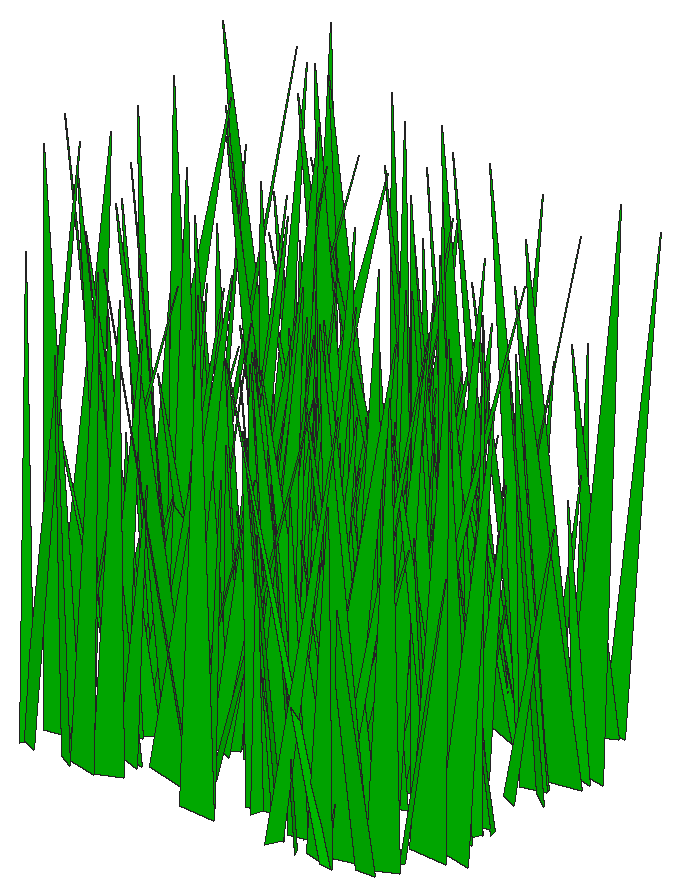
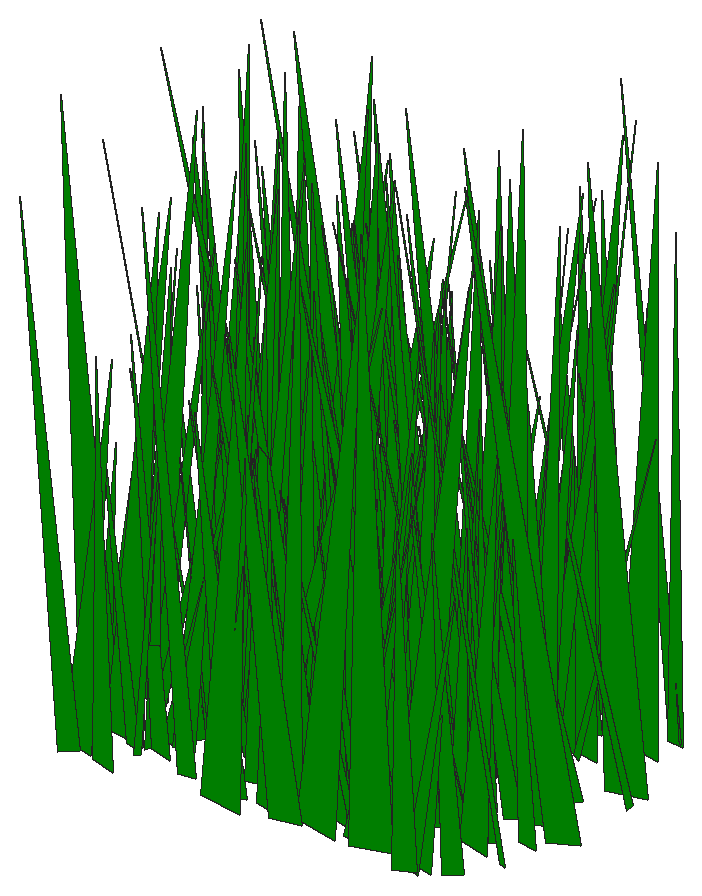
# SketchUp Ruby script. Lengths in inches.
U = 1.inch
M = Sketchup.active_model
def pt(a) = Geom::Point3d.new(a.map { |v| v * U })
def face(e, loops, mat)
  f = e.add_face(loops[0].map { |a| pt(a) })
  loops[1..].each { |l| e.add_face(l.map { |a| pt(a) }).erase! }
  f.material = f.back_material = mat if mat
  f
end
# faces: each face lists its corners as indices into pts; further lists are holes
def faces(e, pts, list, mat = nil) = list.each { |f| face(e, (f[0].is_a?(Array) ? f : [f]).map { |l| l.map { |i| pts[i] } }, mat) }
# xy, xz, yz: faces in a plane at the given z, y or x. An outline is a flat list of corners, or four numbers for a rectangle; further outlines are holes
def ring(l) = l.size == 4 ? [[l[0], l[1]], [l[2], l[1]], [l[2], l[3]], [l[0], l[3]]] : l.each_slice(2).to_a
def flat(e, list, mat, &to3) = list.each { |f| face(e, (f[0].is_a?(Array) ? f : [f]).map { |l| ring(l).map { |u, v| to3.(u, v) } }, mat) }
def xy(e, z, list, mat = nil) = flat(e, list, mat) { |x, y| [x, y, z] }
def xz(e, y, list, mat = nil) = flat(e, list, mat) { |x, z| [x, y, z] }
def yz(e, x, list, mat = nil) = flat(e, list, mat) { |y, z| [x, y, z] }
def lines(e, pts, list) = list.each { |a, b| e.add_line(pt(pts[a]), pt(pts[b])) }
# prism: a flat outline (further loops are holes) pulled along v
def prism(e, loops, v, mat = nil)
  f = face(e, loops, mat); d = Geom::Vector3d.new(v.map { |x| x * U })
  f.pushpull(f.normal.samedirection?(d) ? d.length : -d.length)
end
def box(e, o, s, mat = nil) = prism(e, [[o, [o[0] + s[0], o[1], o[2]], [o[0] + s[0], o[1] + s[1], o[2]], [o[0], o[1] + s[1], o[2]]]], [0, 0, s[2]], mat)
def at(x, y, z, deg = 0) = Geom::Transformation.translation(pt([x, y, z])) * Geom::Transformation.rotation(ORIGIN, Z_AXIS, deg.degrees)
def axes(o, x, y, z) = Geom::Transformation.new([*x, 0, *y, 0, *z, 0, *pt(o).to_a, 1])
def part(name) = M.definitions.add(name)
# library, detail: a bought-in or finely detailed component or shape, given as its bounding box
def library(name, o, s) = part(name).tap { |d| box(d.entities, o, s) }
def detail(e, o, s) = box(e.add_group.entities, o, s)
def put(e, d, t, mat = nil) = e.add_instance(d, t).tap { |i| i.material = mat if mat }
def group(e, t, mat = nil) = e.add_group.tap { |g| g.transformation = t; g.material = mat if mat }.entities
root = M.entities
M.materials.add("[Color G06]").color = [0, 204, 0]
c1 = part("fur_instance\#9")
p = [[0.8125,0,1.79],[0.67,-0.02,1.48],[0,-0.11,0],[0,0.11,0]]
faces(c1.entities,p,[[0,1,2,3]])
put(root,c1,axes([105.97,22.44,4.28],[1.9181,-0.29573,0.60033],[-2.09383,-0.27313,-0.51228],[-0.5242,0.00887,4.2429]),"[Color G06]")
put(root,c1,axes([106.31,16.36,4.28],[-4.10372,0.16999,3.15735],[1.53448,0.62811,0.57038],[1.89584,-0.14044,6.37272]),"[Color G06]")
put(root,c1,axes([106.8,17.14,4.28],[0.83484,0.73798,2.69626],[5.53697,-0.14449,0.71338],[-0.77748,-0.23656,7.97563]),"[Color G06]")
put(root,c1,axes([105.6875,19.02,4.28],[0.77424,-0.81468,1.1639],[-5.87276,-0.09736,0.89807],[0.49908,0.11819,8.76212]),"[Color G06]")
put(root,c1,axes([106.82,20.8,4.28],[4.02849,-0.41541,3.40898],[-3.11493,-0.63045,-0.60285],[-2.09149,0.13881,7.46398]),"[Color G06]")
put(root,c1,axes([107.76,18.34,4.28],[-3.45109,0.03654,0.45566],[0.30965,0.47594,0.85402],[0.2564,-0.08293,5.10177]),"[Color G06]")
put(root,c1,axes([107.32,20.29,4.28],[-3.82285,0.36113,1.39535],[2.57363,0.54791,-0.53947],[0.97712,-0.03028,6.88001]),"[Color G06]")
put(root,c1,axes([106.49,24.64,4.28],[-1.29711,0.40703,1.11347],[2.88676,0.20028,-0.89844],[0.86122,-0.05829,4.68857]),"[Color G06]")
put(root,c1,axes([106.92,23.33,4.28],[0.75746,-0.5353,0.12607],[-3.80054,-0.10623,-0.80832],[-0.5469,-0.00317,5.7918]),"[Color G06]")
put(root,c1,axes([107.39,25.12,4.28],[-1.87838,-0.27256,0.88219],[-2.03753,0.25742,-0.55471],[0.13128,0.09549,4.0134]),"[Color G06]")
put(root,c1,axes([106.375,21.3,4.28],[-0.05739,-0.56329,0.35273],[-4.0176,0.01185,0.71361],[0.48156,0.03173,5.99558]),"[Color G06]")
put(root,c1,axes([107.64,24.82,4.28],[-1.26903,-0.78346,1.78696],[-5.73425,0.16272,-0.90109],[-0.33865,0.18065,8.5614]),"[Color G06]")
put(root,c1,axes([105.22,19.46,4.28],[4.51391,-0.04485,0.29357],[-0.33578,-0.6281,0.50945],[-0.17112,0.0494,6.74426]),"[Color G06]")
put(root,c1,axes([106.25,21.42,4.28],[1.12861,0.45316,1.33911],[3.36202,-0.1417,-0.82095],[0.24603,-0.14248,5.07561]),"[Color G06]")
put(root,c1,axes([105.36,21.84,4.28],[4.11927,-0.60706,1.00444],[-4.40463,-0.56927,0.82644],[-0.05577,0.12111,8.91933]),"[Color G06]")
put(root,c1,axes([106.4,16.27,4.28],[5.39576,0.29573,2.64509],[2.29473,-0.78138,-0.42052],[-1.53758,-0.12835,8.6547]),"[Color G06]")
put(root,c1,axes([107.95,19.875,4.28],[-0.69027,0.49581,1.49692],[3.66458,0.07402,0.95829],[-0.46518,-0.15262,5.32786]),"[Color G06]")
put(root,c1,axes([106.73,22.83,4.28],[4.69642,0.17099,2.31555],[1.4587,-0.67583,-0.8757],[-1.33271,-0.13716,7.2014]),"[Color G06]")
put(root,c1,axes([105.85,23.57,4.28],[5.95394,0.18419,1.47504],[1.38062,-0.83882,-0.41568],[-0.90148,-0.06813,9.10547]),"[Color G06]")
put(root,c1,axes([107.5,25.25,4.28],[-1.10769,0.46629,0.21685],[3.31515,0.15578,-0.65347],[0.46067,0.00013,5.224]),"[Color G06]")
put(root,c1,axes([108.53,18.48,4.28],[-3.92904,0.341,1.49276],[2.56799,0.55158,0.62392],[0.61884,-0.12385,6.88852]),"[Color G06]")
put(root,c1,axes([107.68,16.19,4.28],[3.18649,0.18149,2.81321],[1.63322,-0.49554,-0.4598],[-1.60297,-0.14412,5.1238]),"[Color G06]")
put(root,c1,axes([107.64,23.04,4.28],[-1.09838,-0.38237,0.56293],[-2.73181,0.15885,0.48875],[0.44522,0.03136,4.38771]),"[Color G06]")
put(root,c1,axes([107.05,21.625,4.28],[0.29432,0.37841,0.09989],[2.66708,-0.03857,-0.76957],[0.50498,-0.01684,4.00628]),"[Color G06]")
put(root,c1,axes([106.4,20.08,4.28],[2.59645,-0.26141,0.26695],[-1.87317,-0.35417,0.85626],[0.19341,0.07922,4.70911]),"[Color G06]")
put(root,c1,axes([108.6,17.58,4.28],[-5.70297,-0.19572,2.19023],[-1.35425,0.82108,0.55215],[1.51117,-0.00282,8.76047]),"[Color G06]")
put(root,c1,axes([106.33,21.1,4.28],[3.48903,-0.18994,0.27953],[-1.37447,-0.48008,0.8479],[0.03436,0.08316,5.53332]),"[Color G06]")
put(root,c1,axes([108.5,19.68,4.28],[-5.05139,-0.08644,2.1628],[-0.48664,0.73072,0.81621],[1.49719,-0.05414,7.56239]),"[Color G06]")
put(root,c1,axes([107.78,21.75,4.28],[-1.51105,0.38143,1.10337],[2.74345,0.22612,-0.58694],[0.70736,-0.06219,4.6334]),"[Color G06]")
put(root,c1,axes([107.77,18.14,4.28],[1.12816,-0.61376,0.16786],[-4.37804,-0.15809,-0.67784],[-0.46721,-0.00061,6.75705]),"[Color G06]")
put(root,c1,axes([108.75,23.35,4.28],[-4.65954,0.2701,2.22286],[2.14235,0.66655,0.72732],[1.17221,-0.14456,7.5066]),"[Color G06]")
put(root,c1,axes([108.36,21.43,4.28],[-2.95244,-0.17368,1.08259],[-1.12184,0.42162,0.93614],[0.90412,-0.044,4.69682]),"[Color G06]")
put(root,c1,axes([108.13,21.36,4.28],[-1.51564,-0.38932,0.50522],[-2.76038,0.21618,0.63926],[0.53783,0.01243,4.70468]),"[Color G06]")
put(root,c1,axes([108.24,18.15,4.28],[0.813,0.38856,0.89879],[2.78726,-0.12664,0.65762],[-0.59785,-0.06202,4.28814]),"[Color G06]")
put(root,c1,axes([108.125,20.31,4.28],[3.45609,-0.67049,2.65451],[-4.86621,-0.52304,-1.02432],[-1.61066,0.14152,8.79065]),"[Color G06]")
put(root,c1,axes([108.65,17.29,4.28],[-2.58844,-0.7511,0.59215],[-5.36676,0.36457,0.72007],[0.60625,0.02047,8.90251]),"[Color G06]")
put(root,c1,axes([107.6,23.3125,4.28],[1.85472,0.33706,1.35901],[2.57988,-0.24886,-0.7745],[-0.11644,-0.14504,4.48719]),"[Color G06]")
put(root,c1,axes([107.53,16.53,4.28],[3.17338,0.07105,0.93789],[0.63915,-0.43758,-1.02256],[-0.49488,-0.10953,4.69349]),"[Color G06]")
put(root,c1,axes([109.65,24.8,4.28],[-3.94545,0.00751,0.71812],[0.09413,0.55224,0.49131],[0.47425,-0.04709,5.87681]),"[Color G06]")
put(root,c1,axes([108.22,16.17,4.28],[-2.75667,-0.47668,3.10392],[-3.69131,0.43864,0.41526],[1.54033,0.19808,6.55014]),"[Color G06]")
put(root,c1,axes([109.36,22.81,4.28],[-3.1373,-0.55134,1.69405],[-4.0885,0.43972,-0.47345],[0.44882,0.15171,7.52868]),"[Color G06]")
put(root,c1,axes([107.79,19.47,4.28],[0.91065,-0.45922,1.61291],[-3.44502,-0.10306,0.9739],[0.37629,0.16778,5.01291]),"[Color G06]")
put(root,c1,axes([108.88,21.34,4.28],[-3.51553,0.08603,1.68459],[0.463,0.5119,-0.84481],[1.19862,0.05459,5.26719]),"[Color G06]")
put(root,c1,axes([108.9,22.91,4.28],[1.43097,0.60488,1.82214],[4.39303,-0.22696,0.94855],[-1.00205,-0.13119,6.76058]),"[Color G06]")
put(root,c1,axes([109.31,24.35,4.28],[-3.41214,0.16328,1.57361],[1.33639,0.48559,0.685],[0.83284,-0.11024,5.34791]),"[Color G06]")
put(root,c1,axes([108.8,24.91,4.28],[-1.92857,0.82335,0.8166],[5.87822,0.276,-0.95686],[0.77967,-0.04421,9.23404]),"[Color G06]")
put(root,c1,axes([109.5,18.39,4.28],[-3.31099,-0.63568,0.27825],[-4.51647,0.46121,0.99212],[0.64604,-0.03357,8.36203]),"[Color G06]")
put(root,c1,axes([108.29,17.24,4.28],[1.83773,-0.48935,1.8958],[-3.72187,-0.25452,0.51189],[-0.26767,0.17937,5.89835]),"[Color G06]")
put(root,c1,axes([108.35,23.16,4.28],[-4.42181,0.39574,4.24815],[2.93426,0.72081,-0.89123],[2.74284,-0.13314,7.80201]),"[Color G06]")
put(root,c1,axes([109.7,23.48,4.28],[-3.29177,0.38423,2.27645],[3.0443,0.46681,0.78198],[0.80291,-0.19468,6.36809]),"[Color G06]")
put(root,c1,axes([109.26,18.89,4.28],[0.79037,0.77639,1.09],[5.5915,-0.11826,0.61968],[-0.51616,-0.09222,8.3819]),"[Color G06]")
put(root,c1,axes([109.99,19.21,4.28],[-1.79324,-0.42979,0.62372],[-3.10854,0.24543,-0.5359],[-0.10323,0.07536,5.3024]),"[Color G06]")
put(root,c1,axes([109.8125,23.26,4.28],[-0.06594,-0.36928,1.64454],[-2.80865,-0.02268,-0.83648],[-0.57908,0.15203,3.86982]),"[Color G06]")
put(root,c1,axes([108.91,17.11,4.28],[-0.62293,-0.38489,0.9433],[-2.74508,0.10418,0.83385],[0.69383,0.06662,4.146]),"[Color G06]")
put(root,c1,axes([108.97,16.24,4.28],[2.58087,-0.58388,1.00168],[-4.16704,-0.36949,-0.75839],[-0.78574,0.04166,7.3121]),"[Color G06]")
put(root,c1,axes([107.24,23.03,4.28],[5.58465,0.14579,0.36378],[1.05772,-0.77804,-0.45108],[-0.18331,-0.04764,8.47969]),"[Color G06]")
put(root,c1,axes([108.77,19.15,4.28],[4.06197,-0.25338,1.60984],[-1.74538,-0.58597,-0.75749],[-1.18977,-0.00544,6.60737]),"[Color G06]")
put(root,c1,axes([108.36,18.92,4.28],[3.745,0.35155,1.32375],[2.61446,-0.52601,-0.47457],[-0.55221,-0.10623,6.73057]),"[Color G06]")
put(root,c1,axes([108.02,22.36,4.28],[4.99689,0.26623,1.29252],[2.00453,-0.6981,-0.79225],[-0.61222,-0.11278,7.95543]),"[Color G06]")
put(root,c1,axes([110.01,19.32,4.28],[0.39312,-0.38534,1.31915],[-2.82243,-0.0795,-0.78899],[-0.67022,0.10878,4.09637]),"[Color G06]")
put(root,c1,axes([109.99,19.18,4.28],[0.63779,0.67148,2.06409],[4.95637,-0.11279,0.79392],[-0.72772,-0.17966,7.21624]),"[Color G06]")
put(root,c1,axes([107.99,24.1,4.28],[2.85526,0.62938,0.06828],[4.48492,-0.39474,-0.94303],[0.509,-0.05239,7.92629]),"[Color G06]")
put(root,c1,axes([110.42,24.98,4.28],[-1.29342,-0.7119,2.60973],[-5.39285,0.16258,-0.87562],[-0.17215,0.25571,7.82237]),"[Color G06]")
put(root,c1,axes([108.72,21.25,4.28],[4.82995,-0.2646,1.42997],[-1.86145,-0.6866,-0.55011],[-1.02513,0.00008,7.73626]),"[Color G06]")
put(root,c1,axes([110.93,22.92,4.28],[-2.5487,0.38669,0.55803],[2.79654,0.34969,0.6943],[-0.09298,-0.08209,5.58617]),"[Color G06]")
put(root,c1,axes([109.125,19.41,4.28],[4.05886,0.11811,1.22597],[0.7867,-0.57669,0.56443],[-0.87829,0.02928,6.17119]),"[Color G06]")
put(root,c1,axes([111.42,16.54,4.28],[-4.96307,-0.07387,1.05402],[-0.49246,0.69834,0.44269],[0.73176,-0.03106,7.44666]),"[Color G06]")
put(root,c1,axes([110.17,19.46,4.28],[2.19936,-0.58622,2.48211],[-4.38171,-0.33975,-0.54512],[-1.10997,0.17961,7.07006]),"[Color G06]")
put(root,c1,axes([109.5,24.4,4.28],[2.12057,0.24286,0.80907],[1.80843,-0.29499,-0.41573],[-0.23624,-0.07822,4.08011]),"[Color G06]")
put(root,c1,axes([110.44,23.09,4.28],[-2.66843,0.1725,1.04942],[1.09153,0.38179,-1.00954],[0.91208,0.04778,4.27839]),"[Color G06]")
put(root,c1,axes([109.71,23.41,4.28],[0.48459,-0.51507,0.7046],[-3.70887,-0.06087,0.58665],[0.33131,0.072,5.53677]),"[Color G06]")
put(root,c1,axes([110.26,24.34,4.28],[2.89995,-0.27092,1.74711],[-1.84913,-0.43573,-0.90581],[-1.31216,0.0153,5.13771]),"[Color G06]")
put(root,c1,axes([110.32,19.51,4.28],[-0.96503,-0.41682,0.2855],[-2.96033,0.13699,0.62361],[0.45597,0.00722,4.65295]),"[Color G06]")
put(root,c1,axes([110.71,20.51,4.28],[1.74566,0.42179,1.66019],[3.00418,-0.27675,1.02086],[-1.16531,-0.08161,5.11877]),"[Color G06]")
put(root,c1,axes([109.26,21.52,4.28],[4.74858,-0.27837,1.76883],[-2.13967,-0.67069,0.70597],[-0.8986,0.12599,7.66629]),"[Color G06]")
put(root,c1,axes([110.82,21.88,4.28],[-3.01983,0.29142,0.96141],[1.99617,0.42984,-0.9617],[0.89252,0.02465,5.40383]),"[Color G06]")
put(root,c1,axes([110.13,22.09,4.28],[2.62754,0.02368,1.08578],[0.09455,-0.37846,0.43693],[-0.74004,0.03571,3.91091]),"[Color G06]")
put(root,c1,axes([111.26,21.86,4.28],[-2.82306,0.075,0.89629],[0.46558,0.40062,-0.57512],[0.65736,0.03834,4.25648]),"[Color G06]")
put(root,c1,axes([111.66,22.87,4.28],[-2.03173,-0.76007,1.74599],[-5.57426,0.27564,-0.70526],[-0.04431,0.17558,8.66529]),"[Color G06]")
put(root,c1,axes([109.68,24.45,4.28],[2.88354,0.1677,0.30046],[1.21821,-0.3993,-0.5133],[-0.05194,-0.05502,4.64117]),"[Color G06]")
put(root,c1,axes([110.96,21.39,4.28],[-1.92801,0.56844,1.75764],[4.17336,0.28653,-0.41924],[0.7639,-0.13067,6.72657]),"[Color G06]")
put(root,c1,axes([110.44,19.8,4.28],[2.88864,0.18941,1.73553],[1.61007,-0.40939,-0.85357],[-0.77528,-0.14448,4.69377]),"[Color G06]")
put(root,c1,axes([112.65,24.06,4.28],[-4.24255,-0.40774,0.70701],[-2.96198,0.58478,-0.96099],[0.02004,0.11128,7.64072]),"[Color G06]")
put(root,c1,axes([109.89,18.1,4.28],[3.15194,0.03138,0.31451],[0.18128,-0.43278,0.90252],[-0.24914,0.08213,4.63577]),"[Color G06]")
put(root,c1,axes([111.37,20.08,4.28],[1.8916,0.34284,2.04964],[2.50392,-0.3102,0.79847],[-1.28672,-0.09963,4.56696]),"[Color G06]")
put(root,c1,axes([110.1,17.1,4.28],[2.29045,0.6347,1.52119],[4.66391,-0.31052,-0.80293],[0.03441,-0.16041,7.57305]),"[Color G06]")
put(root,c1,axes([111.65,22.23,4.28],[-1.6296,0.81812,2.11823],[6.03512,0.22376,0.44348],[0.08531,-0.20157,9.08976]),"[Color G06]")
put(root,c1,axes([110.42,20.96,4.28],[1.23671,-0.81607,2.03782],[-5.99667,-0.15517,0.99072],[0.38502,0.20448,8.88477]),"[Color G06]")
put(root,c1,axes([111.31,19.5,4.28],[-1.66949,-0.50049,1.01035],[-3.57815,0.24491,0.72941],[0.73186,0.0557,5.87099]),"[Color G06]")
put(root,c1,axes([110.55,18.92,4.28],[2.67866,-0.08965,0.80296],[-0.74573,-0.3695,0.81805],[-0.38186,0.09275,4.03505]),"[Color G06]")
put(root,c1,axes([111.37,24.81,4.28],[-3.81777,-0.52502,2.74505],[-3.84136,0.57699,0.74324],[1.67119,0.12687,7.97935]),"[Color G06]")
put(root,c1,axes([110.95,24.5,4.28],[0.88865,-0.3734,0.96672],[-2.75228,-0.11634,0.48922],[0.11637,0.09978,4.18821]),"[Color G06]")
put(root,c1,axes([111.5625,18.95,4.28],[-0.77648,-0.57198,0.54023],[-4.10057,0.11209,0.46734],[0.37542,0.04124,6.22182]),"[Color G06]")
put(root,c1,axes([110.46,19.05,4.28],[4.49129,-0.52161,0.75357],[-3.70096,-0.63005,-0.82652],[-0.74092,-0.01468,8.69654]),"[Color G06]")
put(root,c1,axes([111.86,16.14,4.28],[-1.84006,0.64141,1.53205],[4.65818,0.2708,-0.52644],[0.71373,-0.11375,7.38553]),"[Color G06]")
put(root,c1,axes([111.6,20.21,4.28],[-2.50868,0.51104,2.44057],[3.72164,0.39673,-0.99792],[1.49895,-0.12973,6.56228]),"[Color G06]")
put(root,c1,axes([111.24,25.13,4.28],[0.91556,0.6573,0.42097],[4.70856,-0.12405,-0.62406],[0.3571,-0.04953,7.14941]),"[Color G06]")
put(root,c1,axes([111.19,21.65,4.28],[2.7498,-0.11788,0.2941],[-0.79491,-0.37864,-0.83185],[-0.34847,-0.06645,4.21835]),"[Color G06]")
put(root,c1,axes([111.6,19.7,4.28],[-0.61898,0.44944,0.86783],[3.19112,0.10129,-0.94206],[0.73609,-0.0612,4.81377]),"[Color G06]")
put(root,c1,axes([112.01,24.92,4.28],[1.65288,-0.31117,0.95568],[-2.20168,-0.24484,-0.65194],[-0.73557,0.03361,4.09886]),"[Color G06]")
put(root,c1,axes([111.98,16.5,4.28],[2.55938,0.25744,1.24819],[1.72687,-0.37527,0.98196],[-1.06008,0.01022,4.61315]),"[Color G06]")
put(root,c1,axes([111.75,19.67,4.28],[-2.21255,0.4818,2.17808],[3.49569,0.3504,-0.97186],[1.35709,-0.11708,6.05446]),"[Color G06]")
put(root,c1,axes([111.37,20.29,4.28],[4.38019,0.24535,1.62147],[1.71231,-0.62925,0.60529],[-1.1579,-0.00241,7.02892]),"[Color G06]")
put(root,c1,axes([112.6875,18.74,4.28],[-0.90749,-0.53549,1.72642],[-4.00624,0.11379,-0.64937],[-0.17655,0.17032,5.86161]),"[Color G06]")
put(root,c1,axes([112.51,22.96,4.28],[-2.53357,-0.17146,1.05203],[-1.16651,0.36658,0.58787],[0.80407,-0.00843,4.16771]),"[Color G06]")
put(root,c1,axes([111.81,24.09,4.28],[0.05563,0.4103,1.50395],[3.04149,0.02206,-0.94256],[0.64781,-0.13879,4.29624]),"[Color G06]")
put(root,c1,axes([112.75,25.3,4.28],[-3.32769,0.20934,1.60463],[1.43266,0.48758,-0.67062],[1.16357,-0.00165,5.41479]),"[Color G06]")
put(root,c1,axes([112,20.96,4.28],[0.41291,0.6679,2.47819],[5.05823,-0.03948,-0.66044],[0.32389,-0.23499,7.15469]),"[Color G06]")
put(root,c1,axes([111.8125,18.79,4.28],[0.48874,-0.61263,0.19248],[-4.35901,-0.06525,0.86752],[0.56302,0.02665,6.54946]),"[Color G06]")
put(root,c1,axes([111.8125,18.79,4.28],[4.09233,0.22949,1.33408],[1.55192,-0.58316,0.88987],[-1.04723,0.03258,6.532]),"[Color G06]")
put(root,c1,axes([111.39,23.82,4.28],[3.56629,0.47074,1.20213],[3.45504,-0.49669,-0.5526],[-0.32492,-0.11483,7.31847]),"[Color G06]")
put(root,c1,axes([112.97,25.46,4.28],[0.60192,-0.69671,2.7227],[-5.27705,-0.10994,-0.6257],[-0.65917,0.24391,7.49527]),"[Color G06]")
put(root,c1,axes([113.21,17.43,4.28],[-1.34277,0.30325,1.89175],[2.51584,0.1654,0.94318],[0.04519,-0.19712,3.70165]),"[Color G06]")
put(root,c1,axes([112.95,17.23,4.28],[0.71593,-0.46144,1.95975],[-3.51269,-0.12172,-0.42583],[-0.57492,0.16907,5.04217]),"[Color G06]")
put(root,c1,axes([112.6875,19.24,4.28],[3.54295,0.0029,2.09032],[-0.13183,-0.52804,0.58335],[-1.39254,0.05737,5.26307]),"[Color G06]")
put(root,c1,axes([112.9375,24.09,4.28],[-2.51211,-0.50796,1.84932],[-3.68654,0.37676,0.70169],[1.09983,0.10265,6.57603]),"[Color G06]")
put(root,c1,axes([111.26,17.5,4.28],[4.49371,-0.06718,0.19338],[-0.46865,-0.62458,-0.59938],[-0.17091,-0.05371,6.72803]),"[Color G06]")
put(root,c1,axes([112.43,18.42,4.28],[0.11675,-0.66104,2.40701],[-4.97549,0.00969,0.8449],[0.55747,0.22496,7.03667]),"[Color G06]")
put(root,c1,axes([113.45,18.34,4.28],[-2.31426,0.23815,0.64627],[1.67691,0.3283,-0.48357],[0.54,0.00113,4.27139]),"[Color G06]")
put(root,c1,axes([113.62,24.42,4.28],[-4.5737,-0.20862,2.55181],[-1.77727,0.66224,-0.89608],[1.41234,0.15776,7.13611]),"[Color G06]")
put(root,c1,axes([112.35,22.85,4.28],[1.59834,0.3585,1.06482],[2.6666,-0.21122,-0.7717],[0.07983,-0.12219,4.45814]),"[Color G06]")
put(root,c1,axes([112.875,19.93,4.28],[2.86971,-0.09691,1.79877],[-0.9069,-0.42234,0.61797],[-1.0531,0.09963,4.36949]),"[Color G06]")
put(root,c1,axes([113.02,17.08,4.28],[2.22093,-0.22004,1.09577],[-1.47604,-0.32604,-0.8385],[-0.92137,-0.0081,3.98461]),"[Color G06]")
put(root,c1,axes([113.09,22.19,4.28],[1.41464,-0.53262,0.58265],[-3.78771,-0.20308,-0.78294],[-0.62776,0.02507,6.03697]),"[Color G06]")
put(root,c1,axes([112.19,23.9,4.28],[3.23783,0.28922,0.8253],[2.13434,-0.44857,-0.64628],[-0.2264,-0.09257,5.71042]),"[Color G06]")
put(root,c1,axes([112.96,24.99,4.28],[-0.01961,0.55015,0.0047],[3.918,0.00277,-0.69172],[0.46283,-0.00011,5.85581]),"[Color G06]")
put(root,c1,axes([113.88,22.3,4.28],[-0.14578,0.40743,1.22653],[3.0139,0.006,0.57119],[-0.35589,-0.11607,4.33477]),"[Color G06]")
put(root,c1,axes([114.19,16.56,4.28],[-4.10982,-0.19418,1.61934],[-1.25673,0.59099,1.0162],[1.23839,-0.04467,6.40532]),"[Color G06]")
put(root,c1,axes([113.38,22.76,4.28],[1.47615,0.41291,1.98544],[3.23152,-0.20582,-0.44966],[-0.30007,-0.18527,4.92451]),"[Color G06]")
put(root,c1,axes([113.43,20.86,4.28],[-1.37461,-0.51696,1.42523],[-3.70992,0.21473,0.95473],[0.94329,0.09119,5.8318]),"[Color G06]")
put(root,c1,axes([113.125,19.4375,4.28],[1.87645,-0.4373,1.22983],[-3.23932,-0.25841,0.48516],[-0.13531,0.1219,5.44034]),"[Color G06]")
put(root,c1,axes([113.32,20.96,4.28],[2.46556,-0.65761,0.30095],[-4.67954,-0.34469,-0.88545],[-0.61811,-0.01358,7.90396]),"[Color G06]")
put(root,c1,axes([114.5,22.3,4.28],[-4.44381,-0.44776,1.93563],[-3.23449,0.6417,0.4651],[1.23532,0.06946,8.18082]),"[Color G06]")
put(root,c1,axes([114.93,17.28,4.28],[-2.13976,0.54613,0.39643],[3.91598,0.29406,0.67787],[-0.27221,-0.06267,6.63556]),"[Color G06]")
put(root,c1,axes([113.8,21.83,4.28],[4.83263,-0.46303,2.99672],[-3.30618,-0.7253,-0.96404],[-2.02859,0.07903,8.71017]),"[Color G06]")
put(root,c1,axes([114.56,19.17,4.28],[0.84789,0.35071,1.03276],[2.46452,-0.1409,0.9768],[-0.85391,-0.05841,3.84466]),"[Color G06]")
put(root,c1,axes([114.625,23.03,4.28],[1.0786,-0.34461,1.50115],[-2.51546,-0.18168,-0.75382],[-0.88797,0.09608,3.95883]),"[Color G06]")
put(root,c1,axes([114.375,21.15,4.28],[1.94143,0.5475,2.13278],[4.07928,-0.29577,0.42761],[-0.9009,-0.1594,6.53234]),"[Color G06]")
put(root,c1,axes([116.02,16.02,4.28],[-4.71552,0.135,0.3314],[0.94712,0.6564,-0.6123],[0.2989,0.04982,7.16858]),"[Color G06]")
put(root,c1,axes([114.58,16.75,4.28],[0.86598,0.41911,1.38681],[3.08795,-0.13883,0.51233],[-0.59894,-0.10978,4.64656]),"[Color G06]")
put(root,c1,axes([113.57,22.29,4.28],[3.14288,-0.284,1.32386],[-2.17599,-0.4366,0.77984],[-0.44451,0.12926,5.5427]),"[Color G06]")
put(root,c1,axes([114.95,21.52,4.28],[1.6294,0.69313,2.45859],[5.10014,-0.26445,1.01424],[-1.18407,-0.18523,7.7519]),"[Color G06]")
put(root,c1,axes([115.03,16.11,4.28],[2.92169,0.11244,2.6138],[0.56344,-0.47365,0.93375],[-1.84153,0.03347,4.43264]),"[Color G06]")
put(root,c1,axes([115.1875,21.77,4.28],[-0.07094,0.71294,1.82216],[5.21443,-0.0118,0.9837],[-0.65979,-0.16989,7.57839]),"[Color G06]")
put(root,c1,axes([113.15,20.33,4.28],[4.69786,0.201,0.55373],[1.39413,-0.65421,0.85989],[-0.521,0.06187,7.29387]),"[Color G06]")
put(root,c1,axes([115.33,23.92,4.28],[-4.28341,-0.49489,1.71422],[-3.53213,0.61647,0.72982],[1.19789,0.04811,8.28168]),"[Color G06]")
put(root,c1,axes([114.0625,17.55,4.28],[3.27799,0.59329,0.57428],[4.20363,-0.46,0.99396],[-0.76087,0.01463,7.9655]),"[Color G06]")
put(root,c1,axes([113.81,23.35,4.28],[3.22784,-0.13971,0.21581],[-0.95762,-0.44327,-0.97063],[-0.32803,-0.08071,4.95716]),"[Color G06]")
put(root,c1,axes([115.87,23.84,4.28],[-2.83836,0.1381,0.53192],[1.03861,0.39061,0.73006],[0.16952,-0.08089,4.43323]),"[Color G06]")
put(root,c1,axes([114.97,22.03,4.28],[-4.35024,0.30166,3.57654],[2.52842,0.66676,0.40945],[2.00332,-0.18648,7.24971]),"[Color G06]")
put(root,c1,axes([114.86,21.12,4.28],[3.12168,0.1679,1.61871],[1.1085,-0.46062,0.71314],[-1.18065,0.01146,4.94948]),"[Color G06]")
put(root,c1,axes([114.5,19.37,4.28],[2.61897,0.19289,1.49664],[1.62514,-0.36005,-1.02162],[-0.52456,-0.15243,4.30719]),"[Color G06]")
put(root,c1,axes([114.47,24.87,4.28],[4.16783,0.36988,2.40763],[2.89344,-0.59914,-0.61465],[-1.12206,-0.17108,7.35805]),"[Color G06]")
put(root,c1,axes([115.78,21.02,4.28],[-2.87339,0.09362,1.13603],[0.80012,0.40495,0.68714],[0.62311,-0.08829,4.35629]),"[Color G06]")
put(root,c1,axes([114.83,23.59,4.28],[2.65233,0.05307,1.09079],[0.22552,-0.37709,0.88271],[-0.79161,0.07039,3.9062]),"[Color G06]")
put(root,c1,axes([115.59,19.4,4.28],[-0.05913,0.46949,0.03336],[3.34412,0.00783,0.58485],[-0.39087,-0.00405,4.99862]),"[Color G06]")
put(root,c1,axes([115.27,23.1875,4.28],[-3.48263,0.25175,2.12355],[1.72741,0.52416,-0.81011],[1.51464,-0.01894,5.80661]),"[Color G06]")
put(root,c1,axes([114.9,17.36,4.28],[-0.31879,-0.54139,1.26011],[-3.93504,0.05929,0.70233],[0.54768,0.11083,5.77966]),"[Color G06]")
put(root,c1,axes([116.16,16.79,4.28],[-2.91319,0.12861,0.2971],[0.86733,0.40047,-0.91749],[0.37133,0.07359,4.47386]),"[Color G06]")
put(root,c1,axes([115.19,20.11,4.28],[2.33871,-0.35423,1.32088],[-2.55674,-0.34349,-0.47007],[-0.83496,0.05963,5.13917]),"[Color G06]")
put(root,c1,axes([114.28,16.17,4.28],[4.22542,-0.29334,0.59632],[-2.04547,-0.58941,-0.93155],[-0.63282,-0.0535,6.99277]),"[Color G06]")
put(root,c1,axes([114.32,18.74,4.28],[1.93018,-0.33175,0.00395],[-2.34104,-0.26477,0.8184],[0.42359,0.04839,4.50501]),"[Color G06]")
put(root,c1,axes([114.92,19.91,4.28],[2.75299,-0.34878,0.5535],[-2.46435,-0.38721,-0.64913],[-0.56573,-0.01056,5.52108]),"[Color G06]")
put(root,c1,axes([116.59,23.43,4.28],[-2.91181,0.15197,0.41989],[1.11403,0.40464,0.4326],[0.1601,-0.05163,4.62658]),"[Color G06]")
put(root,c1,axes([114.85,20.05,4.28],[4.61273,-0.24887,1.70735],[-1.72787,-0.66265,-0.66835],[-1.22665,-0.00244,7.36182]),"[Color G06]")
put(root,c1,axes([116.02,24.28,4.28],[-2.6851,0.25891,0.98895],[1.73696,0.38451,-1.02975],[0.93183,0.02933,4.76921]),"[Color G06]")
put(root,c1,axes([116.05,24.8,4.28],[-2.37304,-0.18748,1.01094],[-1.28396,0.34407,0.5976],[0.78523,-0.00399,4.03232]),"[Color G06]")
put(root,c1,axes([115.13,19.49,4.28],[2.92964,0.13015,0.55552],[0.85153,-0.40649,0.90851],[-0.53302,0.06593,4.50469]),"[Color G06]")
put(root,c1,axes([116.67,16.75,4.28],[-1.32093,0.70204,1.00652],[5.07221,0.17716,0.67411],[-0.26964,-0.10659,7.74989]),"[Color G06]")
put(root,c1,axes([114.87,16.94,4.28],[3.42998,-0.2799,0.13862],[-1.9703,-0.47352,-0.9323],[-0.3942,-0.06864,5.86599]),"[Color G06]")
put(root,c1,axes([115.54,22.09,4.28],[3.32982,0.22789,2.0784],[1.89852,-0.47972,-0.7519],[-1.00013,-0.15191,5.4925]),"[Color G06]")
put(root,c1,axes([115.31,19.27,4.28],[2.49805,-0.51069,2.05459],[-3.89605,-0.34522,0.72391],[-0.35106,0.19726,6.58602]),"[Color G06]")
put(root,c1,axes([115.75,16.14,4.28],[-0.70227,-0.51113,0.62415],[-3.63567,0.10595,0.82906],[0.62592,0.04191,5.51595]),"[Color G06]")
put(root,c1,axes([117.01,16.39,4.28],[-3.1876,-0.42432,1.37135],[-3.14775,0.44652,-0.47243],[0.43904,0.12069,6.56933]),"[Color G06]")
put(root,c1,axes([116.91,23.0625,4.28],[-3.90641,-0.37598,0.97196],[-2.62695,0.55181,0.93685],[0.88993,-0.02155,7.03197]),"[Color G06]")
put(root,c1,axes([115.47,16.77,4.28],[2.73008,0.19866,0.50583],[1.37137,-0.38189,0.69566],[-0.51323,0.03631,4.54955]),"[Color G06]")
put(root,c1,axes([116.37,16.57,4.28],[0.60744,-0.78152,0.40623],[-5.58491,-0.08789,-0.76899],[-0.54129,0.02978,8.39022]),"[Color G06]")
put(root,c1,axes([115.42,21.24,4.28],[3.91476,-0.43972,2.31262],[-3.38615,-0.55832,0.60898],[-0.93363,0.1812,7.48821]),"[Color G06]")
put(root,c1,axes([115.61,24.45,4.28],[3.20829,-0.30748,0.88899],[-2.13133,-0.45449,-0.87627],[-0.82055,-0.02172,5.75196]),"[Color G06]")
put(root,c1,axes([116.38,19.66,4.28],[1.70699,-0.63358,2.29116],[-4.69509,-0.26696,-0.66669],[-0.97477,0.17632,7.22342]),"[Color G06]")
put(root,c1,axes([116.09,22.01,4.28],[-0.39044,0.38527,1.33294],[2.83716,0.07726,-0.70878],[0.61595,-0.11163,4.10967]),"[Color G06]")
put(root,c1,axes([116.8125,24.34,4.28],[0.01302,-0.7359,0.40761],[-5.27155,-0.00446,-0.54835],[-0.36806,0.03781,7.86832]),"[Color G06]")
put(root,c1,axes([116.86,20.86,4.28],[1.22644,-0.50457,2.68025],[-3.92357,-0.21076,-0.54742],[-0.95622,0.21763,5.68385]),"[Color G06]")
put(root,c1,axes([116.36,25.73,4.28],[2.8801,-0.34226,1.23802],[-2.36184,-0.4179,-0.99835],[-1.06409,0.00117,5.5668]),"[Color G06]")
put(root,c1,axes([117.46,22.48,4.28],[-4.19624,0.56599,1.59665],[4.08115,0.59941,-0.45012],[0.97971,-0.07274,8.71377]),"[Color G06]")
put(root,c1,axes([117.68,18.72,4.28],[-1.84378,0.48811,0.36209],[3.50123,0.25344,0.57709],[-0.2299,-0.05489,5.88475]),"[Color G06]")
put(root,c1,axes([115.1875,23.12,4.28],[5.46856,0.06772,1.05599],[0.41074,-0.76529,0.88686],[-0.75258,0.07444,8.15727]),"[Color G06]")
put(root,c1,axes([115.45,16.79,4.28],[2.49758,-0.72061,0.12231],[-5.15761,-0.3467,0.61036],[0.33221,0.03503,8.55645]),"[Color G06]")
put(root,c1,axes([116.35,24.58,4.28],[2.43972,-0.2207,0.36192],[-1.5277,-0.3393,-0.76408],[-0.47918,-0.04192,4.27869]),"[Color G06]")
put(root,c1,axes([117.39,25.42,4.28],[0.66991,-0.49617,1.66192],[-3.63569,-0.12178,-0.90308],[-0.82404,0.13394,5.33554]),"[Color G06]")
put(root,c1,axes([117.34,18.58,4.28],[2.30377,0.15752,1.99308],[1.0451,-0.37077,0.66786],[-1.40077,-0.01756,3.77619]),"[Color G06]")
put(root,c1,axes([115.79,16.59,4.28],[5.3854,-0.13384,1.33112],[-1.05475,-0.75493,0.81242],[-0.77585,0.09729,8.13524]),"[Color G06]")
put(root,c1,axes([117.64,22.25,4.28],[0.62315,0.54689,1.82255],[4.05166,-0.11002,0.69816],[-0.67263,-0.15608,5.89389]),"[Color G06]")
put(root,c1,axes([115.24,19.75,4.28],[5.71636,-0.16368,0.52881],[-1.19447,-0.79658,0.51863],[-0.27605,0.05739,8.70634]),"[Color G06]")
put(root,c1,axes([117.93,19.65,4.28],[-2.15691,-0.27455,1.26088],[-2.10877,0.30146,-0.51733],[0.37579,0.11586,4.33396]),"[Color G06]")
put(root,c1,axes([117.61,19.22,4.28],[2.57719,0.55752,4.68737],[4.90047,-0.40239,-0.52057],[-1.34399,-0.39812,7.09023]),"[Color G06]")
put(root,c1,axes([117.78,19.97,4.28],[0.22349,0.41034,1.65475],[3.11309,-0.05054,0.50059],[-0.44001,-0.14917,4.38216]),"[Color G06]")
put(root,c1,axes([118.12,22.89,4.28],[-0.77761,-0.69909,0.50954],[-5.01494,0.10493,-0.55702],[-0.31701,0.05484,7.56196]),"[Color G06]")
put(root,c1,axes([118.22,19.92,4.28],[-2.66248,-0.08887,0.98274],[-0.7907,0.36531,-0.99038],[0.46182,0.11313,3.97001]),"[Color G06]")
put(root,c1,axes([117.31,16.71,4.28],[2.19834,-0.65861,0.12736],[-4.68329,-0.30558,-0.95922],[-0.61763,-0.02708,7.72684]),"[Color G06]")
put(root,c1,axes([118.09,21.97,4.28],[-3.79056,-0.20977,1.66733],[-1.38874,0.55045,0.90315],[1.25656,-0.02445,6.02782]),"[Color G06]")
put(root,c1,axes([118.26,23.39,4.28],[-1.60757,0.32517,0.05439],[2.30538,0.2225,-0.60254],[0.35239,0.02778,4.18998]),"[Color G06]")
put(root,c1,axes([117.7,18,4.28],[1.3214,-0.64314,2.64895],[-4.9371,-0.18202,0.42463],[-0.19613,0.24881,7.15797]),"[Color G06]")
put(root,c1,axes([117.44,17.3,4.28],[2.76657,0.15288,0.67433],[1.04614,-0.38996,0.56846],[-0.55774,0.02688,4.41117]),"[Color G06]")
put(root,c1,axes([117.4375,25.7,4.28],[4.23447,-0.32353,2.3034],[-2.5552,-0.60687,0.70078],[-1.1087,0.16297,7.18235]),"[Color G06]")
put(root,c1,axes([117.99,19.52,4.28],[-4.30015,0.13052,3.56498],[1.34541,0.66801,0.81556],[2.18071,-0.15477,6.52661]),"[Color G06]")
put(root,c1,axes([117.5,21.47,4.28],[2.28238,0.22805,0.88164],[1.72054,-0.31577,-0.56658],[-0.24949,-0.09138,4.15806]),"[Color G06]")
put(root,c1,axes([118.13,23.64,4.28],[-1.35726,0.70191,3.31701],[5.35926,0.24064,-0.95121],[1.24133,-0.27146,7.73348]),"[Color G06]")
put(root,c1,axes([118.22,18.31,4.28],[-0.0594,0.5992,2.01343],[4.45062,0.03644,-0.95255],[0.68627,-0.18447,6.35176]),"[Color G06]")
